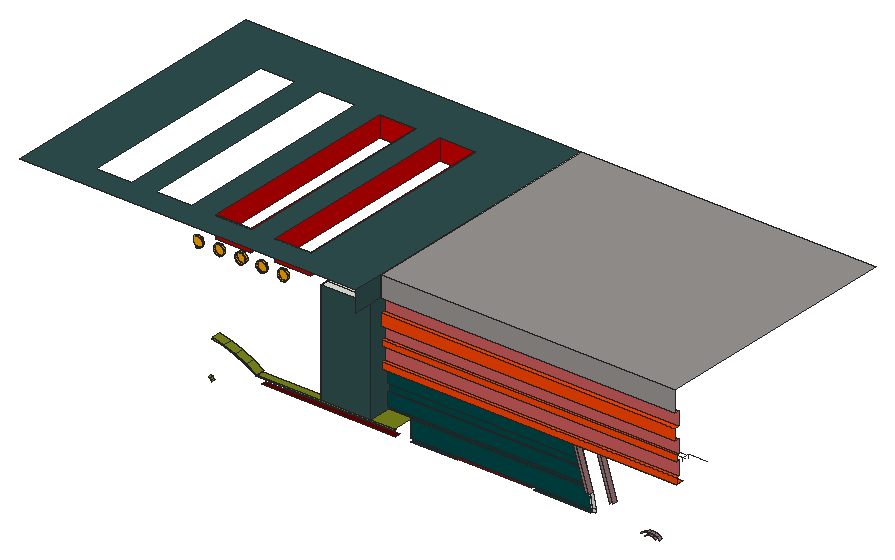
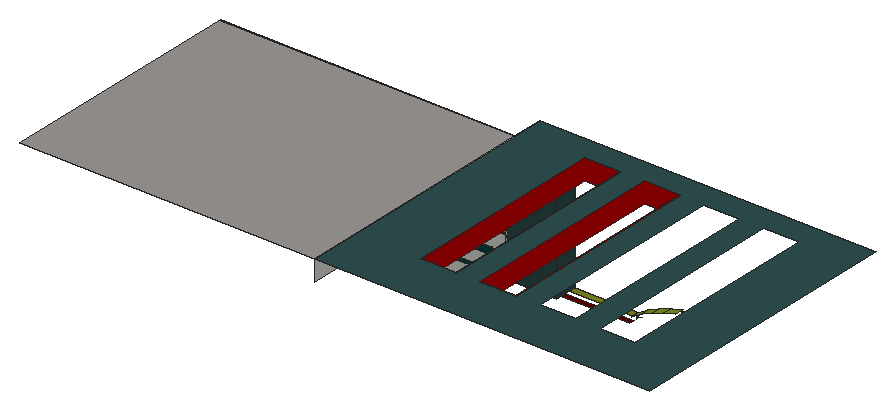
# SketchUp Ruby script. Lengths in inches.
U = 1.inch
M = Sketchup.active_model
def pt(a) = Geom::Point3d.new(a.map { |v| v * U })
def face(e, loops, mat)
  f = e.add_face(loops[0].map { |a| pt(a) })
  loops[1..].each { |l| e.add_face(l.map { |a| pt(a) }).erase! }
  f.material = f.back_material = mat if mat
  f
end
# faces: each face lists its corners as indices into pts; further lists are holes
def faces(e, pts, list, mat = nil) = list.each { |f| face(e, (f[0].is_a?(Array) ? f : [f]).map { |l| l.map { |i| pts[i] } }, mat) }
# xy, xz, yz: faces in a plane at the given z, y or x. An outline is a flat list of corners, or four numbers for a rectangle; further outlines are holes
def ring(l) = l.size == 4 ? [[l[0], l[1]], [l[2], l[1]], [l[2], l[3]], [l[0], l[3]]] : l.each_slice(2).to_a
def flat(e, list, mat, &to3) = list.each { |f| face(e, (f[0].is_a?(Array) ? f : [f]).map { |l| ring(l).map { |u, v| to3.(u, v) } }, mat) }
def xy(e, z, list, mat = nil) = flat(e, list, mat) { |x, y| [x, y, z] }
def xz(e, y, list, mat = nil) = flat(e, list, mat) { |x, z| [x, y, z] }
def yz(e, x, list, mat = nil) = flat(e, list, mat) { |y, z| [x, y, z] }
def lines(e, pts, list) = list.each { |a, b| e.add_line(pt(pts[a]), pt(pts[b])) }
# prism: a flat outline (further loops are holes) pulled along v
def prism(e, loops, v, mat = nil)
  f = face(e, loops, mat); d = Geom::Vector3d.new(v.map { |x| x * U })
  f.pushpull(f.normal.samedirection?(d) ? d.length : -d.length)
end
def box(e, o, s, mat = nil) = prism(e, [[o, [o[0] + s[0], o[1], o[2]], [o[0] + s[0], o[1] + s[1], o[2]], [o[0], o[1] + s[1], o[2]]]], [0, 0, s[2]], mat)
def at(x, y, z, deg = 0) = Geom::Transformation.translation(pt([x, y, z])) * Geom::Transformation.rotation(ORIGIN, Z_AXIS, deg.degrees)
def axes(o, x, y, z) = Geom::Transformation.new([*x, 0, *y, 0, *z, 0, *pt(o).to_a, 1])
def part(name) = M.definitions.add(name)
# library, detail: a bought-in or finely detailed component or shape, given as its bounding box
def library(name, o, s) = part(name).tap { |d| box(d.entities, o, s) }
def detail(e, o, s) = box(e.add_group.entities, o, s)
def put(e, d, t, mat = nil) = e.add_instance(d, t).tap { |i| i.material = mat if mat }
def group(e, t, mat = nil) = e.add_group.tap { |g| g.transformation = t; g.material = mat if mat }.entities
root = M.entities
M.materials.add("[0017_IndianRed]").color = [205, 92, 92]
M.materials.add("[0020_Red]").color = [165, 0, 0]
M.materials.add("[0020_Red]1").color = [204, 0, 0]
M.materials.add("[0022_Maroon]").color = [99, 0, 0]
M.materials.add("[0024_OrangeRed]").color = [255, 69, 0]
M.materials.add("[0038_Orange]1").color = [255, 165, 0]
M.materials.add("[0057_DarkKhaki]").color = [122, 132, 27]
M.materials.add("[0078_DarkSlateGray]").color = [47, 79, 79]
M.materials.add("[0119_RosyBrown]").color = [150, 114, 114]
M.materials.add("[Color H08]").color = [0, 71, 71]
M.materials.add("[Concrete Aggregate Smoke]").color = [154, 150, 148]
xy(root,288.67,[[221.0625,650.11,247.97,651.11],[292.45,650.11,325.55,651.11]],"[Color H08]")
xy(root,290.61,[[247.97,650.11,292.45,651.11],[247.97,651.11,292.45,656.36]])
xy(root,290.61,[[247.97,648.11,292.45,650.11]],"[0020_Red]")
xy(root,290.61,[[221.0625,650.11,247.97,651.11],[292.45,650.11,325.22,651.11]],"[Color H08]")
xy(root,296.25,[[143.09,639.11,221.0625,642.11]],"[0022_Maroon]")
xy(root,299.9,[[140.36,638.11,221.0625,639.11]],"[0057_DarkKhaki]")
xy(root,300.74,[[178.3125,638.05,207.0625,638.11],[178.3125,638.11,207.0625,642.11],[178.3125,642.11,178.3125,651.24,207.9375,651.24,207.9375,651.11,207.0625,651.11,207.0625,642.11],[207.9375,651.11,221.0625,651.24]])
xy(root,300.74,[[141.15,638.11,178.3125,642.11],[207.0625,638.11,221.0625,651.11]],"[0057_DarkKhaki]")
xy(root,300.74,[[221.0625,650.11,323.2,651.11]],"[Color H08]")
xy(root,302.39,[[207.0625,650.11,207.9375,651.11]])
xy(root,302.39,[[207.9375,650.11,322.69,651.11]],"[Color H08]")
xy(root,310.14,[[207.0625,650.11,320.31,651.11]],"[Color H08]")
xy(root,314.28,[[207.0625,650.11,319.04,651.11]],"[Color H08]")
xy(root,323.31,[[316.26,648.11,317.96,651.11],[207.9375,650.11,316.26,651.11]])
xy(root,323.31,[[207.0625,646.43,207.0625,650.11,316.26,650.11,316.26,648.11,317.96,648.11,317.96,651.11,330.34,651.11,330.34,648.11,332.04,648.11,332.04,651.11,377.9375,651.11,377.9375,646.43]],"[0024_OrangeRed]")
xy(root,326.96,[[207.0625,646.43,377.9375,648.43]],"[0024_OrangeRed]")
xy(root,335.1875,[[207.0625,646.43,377.9375,648.43]],"[0024_OrangeRed]")
xy(root,338.52,[[207.0625,646.43,377.9375,648.43]],"[0024_OrangeRed]")
xy(root,346.17,[[207.0625,645.43,377.9375,648.43]],"[0024_OrangeRed]")
xy(root,352.6875,[[207.0625,645.43,377.9375,648.43]],"[0024_OrangeRed]")
xy(root,360.74,[[178.3125,638.05,207,638.11],[207,638.05,207.0625,645.43],[178.3125,638.11,207,642.11],[178.3125,642.11,207,651.24],[207,645.43,207.0625,645.43,207.0625,648.43,207.9375,648.43,207.9375,651.24,207,651.24]])
xy(root,360.74,[[207.0625,645.43,377.9375,648.43]],"[Concrete Aggregate Smoke]")
xy(root,372.74,[[[12.25,627.18,207,791.05],[45.02,641.59,65.77,760.78],[79.64,641.59,100.39,760.78],[114.27,641.59,135.02,760.78],[148.89,641.59,169.64,760.78]]],"[0078_DarkSlateGray]")
xy(root,372.74,[[207,645.43,377.9375,791.05]],"[Concrete Aggregate Smoke]")
xz(root,628.18,[[115.26,362.59,116.05,362.69,116.79,363,117.42,363.48,117.91,364.12,118.22,364.86,118.32,365.65,118.22,366.44,117.91,367.18,117.42,367.82,116.79,368.3,116.05,368.61,115.26,368.71,114.47,368.61,113.73,368.3,113.09,367.82,112.61,367.18,112.3,366.44,112.2,365.65,112.3,364.86,112.61,364.12,113.09,363.48,113.73,363,114.47,362.69],[127.63,362.59,128.43,362.69,129.16,363,129.8,363.48,130.29,364.12,130.59,364.86,130.7,365.65,130.59,366.44,130.29,367.18,129.8,367.82,129.16,368.3,128.43,368.61,127.63,368.71,126.84,368.61,126.1,368.3,125.47,367.82,124.98,367.18,124.68,366.44,124.57,365.65,124.68,364.86,124.98,364.12,125.47,363.48,126.1,363,126.84,362.69],[152.38,362.59,153.18,362.69,153.91,363,154.55,363.48,155.04,364.12,155.34,364.86,155.45,365.65,155.34,366.44,155.04,367.18,154.55,367.82,153.91,368.3,153.18,368.61,152.38,368.71,151.59,368.61,150.85,368.3,150.22,367.82,149.73,367.18,149.43,366.44,149.32,365.65,149.43,364.86,149.73,364.12,150.22,363.48,150.85,363,151.59,362.69],[164.76,362.59,165.55,362.69,166.29,363,166.92,363.48,167.41,364.12,167.72,364.86,167.82,365.65,167.72,366.44,167.41,367.18,166.92,367.82,166.29,368.3,165.55,368.61,164.76,368.71,163.97,368.61,163.23,368.3,162.59,367.82,162.11,367.18,161.8,366.44,161.7,365.65,161.8,364.86,162.11,364.12,162.59,363.48,163.23,363,163.97,362.69]],"[0038_Orange]1")
xz(root,628.86,[[140.01,362.59,140.8,362.69,141.54,363,142.17,363.48,142.66,364.12,142.97,364.86,143.07,365.65,142.97,366.44,142.66,367.18,142.17,367.82,141.54,368.3,140.8,368.61,140.01,368.71,139.22,368.61,138.48,368.3,137.84,367.82,137.36,367.18,137.05,366.44,136.95,365.65,137.05,364.86,137.36,364.12,137.84,363.48,138.48,363,139.22,362.69]],"[0038_Orange]1")
xz(root,638.05,[[178.3125,300.74,207.0625,360.74]],"[0078_DarkSlateGray]")
xz(root,641.59,[[114.27,360.74,135.02,372.74],[148.89,360.74,169.64,372.74]],"[0020_Red]1")
xz(root,642.11,[[138.39,300.67,141.15,300.6875],[138.39,300.6875,138.39,300.74,138.48,300.6875],[138.48,300.6875,138.39,300.74,141.15,300.74,141.15,300.6875]])
xz(root,645.43,[[207.0625,346.17,377.9375,352.6875]],"[0024_OrangeRed]")
xz(root,645.43,[[207,360.74,377.9375,372.74]],"[Concrete Aggregate Smoke]")
xz(root,646.43,[[207.0625,323.31,377.9375,326.96],[207.0625,335.1875,377.9375,338.52]],"[0024_OrangeRed]")
xz(root,648.43,[[207.9375,335.1875,367,338.52]])
xz(root,648.43,[[207.0625,326.96,377.9375,335.1875],[207.0625,338.52,377.9375,346.17],[207.0625,352.6875,377.9375,360.74]],"[0017_IndianRed]")
xz(root,650.11,[[221.0625,290.61,325.22,290.61,323.87,298.58,323.2,300.74,221.0625,300.74],[207.0625,302.39,322.69,302.39,320.31,310.14,207.0625,310.14],[207.0625,314.28,319.04,314.28,316.26,323.31,207.0625,323.31]],"[Color H08]")
xz(root,651.11,[[325.55,288.67,327.54,288.67,327.19,290.61,325.22,290.61],[221.0625,290.61,221.0625,300.74,323.2,300.74,323.87,298.58,325.22,290.61],[325.22,290.61,327.19,290.61,325.7,298.89,325.11,300.74,323.2,300.74,323.87,298.58],[323.2,300.74,325.11,300.74,324.59,302.39,322.69,302.39],[207.9375,302.39,207.9375,310.14,320.31,310.14,322.69,302.39],
  [322.69,302.39,324.59,302.39,322.13,310.14,320.31,310.14],[320.31,310.14,322.13,310.14,319.04,319.9,319.04,314.28],[207.9375,314.28,207.9375,323.31,316.26,323.31,319.04,314.28],[319.04,314.28,319.04,319.9,317.96,323.31,316.26,323.31]])
xz(root,651.11,[[221.0625,288.67,247.97,290.61],[292.45,288.67,325.55,288.67,325.22,290.61,292.45,290.61],[207.0625,300.74,323.2,300.74,322.69,302.39,207.0625,302.39],[207.0625,310.14,320.31,310.14,319.04,314.28,207.0625,314.28]],"[Color H08]")
xz(root,651.24,[[207,300.74,207.9375,360.74]])
xz(root,651.24,[[178.3125,300.74,207,360.74]],"[0078_DarkSlateGray]")
xz(root,760.78,[[114.27,360.74,135.02,372.74],[148.89,360.74,169.64,372.74]],"[0020_Red]1")
yz(root,114.27,[[641.59,360.74,760.78,372.74]],"[0020_Red]1")
yz(root,135.02,[[641.59,360.74,760.78,372.74]],"[0020_Red]1")
yz(root,140.36,[[638.11,299.9,639.11,300.29]],"[0057_DarkKhaki]")
yz(root,141.15,[[639.11,300.67,642.11,300.6875],[642.11,300.67,643.36,300.6875],[639.11,300.6875,642.11,300.74],[642.11,300.6875,643.36,300.74]])
yz(root,148.89,[[641.59,360.74,760.78,372.74]],"[0020_Red]1")
yz(root,169.64,[[641.59,360.74,760.78,372.74]],"[0020_Red]1")
yz(root,178.3125,[[638.05,300.74,651.24,360.74]],"[0078_DarkSlateGray]")
yz(root,207,[[645.43,360.74,791.05,372.74]])
yz(root,207,[[627.18,360.74,645.43,372.74]],"[0078_DarkSlateGray]")
yz(root,207.0625,[[638.05,300.74,651.11,300.74,651.11,302.39,650.11,302.39,650.11,310.14,651.11,310.14,651.11,314.28,650.11,314.28,650.11,323.31,646.43,323.31,646.43,326.96,648.43,326.96,648.43,335.1875,646.43,335.1875,646.43,338.52,648.43,338.52,648.43,346.17,645.43,346.17,645.43,352.6875,648.43,352.6875,648.43,360.74,638.05,360.74]],"[0078_DarkSlateGray]")
yz(root,221.0625,[[650.11,290.61,651.11,300.74]])
yz(root,247.97,[[651.11,288.67,656.36,290.61]])
yz(root,292.45,[[651.11,288.67,656.36,290.61]])
p = [[357.6875,651.11,288.52],[359.11,651.11,289.11],[359.11,649.11,289.11],[357.6875,649.11,288.52],[362.16,651.11,289.11],[363.58,651.11,288.52],
  [363.58,649.11,288.52],[362.16,649.11,289.11],[115.7,639.11,288.64],[115.4,639.11,289.31],[115.4,637.11,289.31],[115.7,637.11,288.64],
  [356.85,651.11,289.97],[355.29,651.11,288.77],[355.29,649.11,288.77],[356.85,649.11,289.97],[365.98,651.11,288.77],[364.42,651.11,289.97],
  [364.42,649.11,289.97],[365.98,649.11,288.77],[360.63,651.11,289.3125],[360.63,649.11,289.3125],[114.97,639.11,289.9],[114.97,637.11,289.9],
  [114.43,639.11,290.38],[114.43,637.11,290.38],[358.68,651.11,290.72],[358.68,649.11,290.72],[362.59,651.11,290.72],[362.59,649.11,290.72],
  [113.8,639.11,290.75],[113.8,637.11,290.75],[323.87,651.11,298.58],[325.22,651.11,290.61],[325.22,650.11,290.61],[323.87,650.11,298.58],
  [360.63,651.11,290.98],[360.63,649.11,290.98],[322.69,651.11,302.39],[323.2,651.11,300.74],[323.2,650.11,300.74],[323.87,648.11,298.58],
  [316.26,648.11,323.31],[316.26,650.11,323.31],[319.04,650.11,314.28],[319.04,651.11,314.28],[320.31,651.11,310.14],[320.31,650.11,310.14],
  [322.69,650.11,302.39],[330.34,651.11,323.31],[337.94,651.11,298.58],[337.94,648.11,298.58],[330.34,648.11,323.31],[325.7,651.11,298.89],
  [325.11,651.11,300.74],[324.59,651.11,302.39],[322.13,651.11,310.14],[319.04,651.11,319.9],[317.96,651.11,323.31],[317.96,648.11,323.31],
  [325.7,648.11,298.89],[339.78,651.11,298.89],[332.04,651.11,323.31],[332.04,648.11,323.31],[339.78,648.11,298.89],[134.72,639.11,303.6],
  [140.36,639.11,300.29],[140.36,638.11,300.29],[134.72,638.11,303.6],[135.09,643.36,304.29],[135.09,638.11,304.29],[141.15,638.11,300.74],
  [141.15,639.11,300.74],[141.15,642.11,300.74],[141.15,643.36,300.74],[128.42,639.11,306.52],[128.42,638.11,306.52],[128.71,643.36,307.25],
  [128.71,638.11,307.25],[121.85,639.11,308.82],[121.85,638.11,308.82],[122.08,643.36,309.58],[122.08,638.11,309.58],[115.1,639.11,310.48],
  [115.1,638.11,310.48],[115.25,643.36,311.26],[115.25,638.11,311.26],[316.26,651.11,323.31],[114.47,627.18,362.69],[115.26,627.18,362.59],
  [115.26,628.18,362.59],[114.47,628.18,362.69],[116.05,627.18,362.69],[116.05,628.18,362.69],[126.84,627.18,362.69],[127.63,627.18,362.59],
  [127.63,628.18,362.59],[126.84,628.18,362.69],[128.43,627.18,362.69],[128.43,628.18,362.69],[139.22,627.18,362.69],[140.01,627.18,362.59],
  [140.01,627.24,362.59],[139.22,627.24,362.69],[139.22,628.86,362.69],[140.01,628.86,362.59],[140.8,627.18,362.69],[140.8,627.24,362.69],
  [140.8,628.86,362.69],[151.59,627.18,362.69],[152.38,627.18,362.59],[152.38,628.18,362.59],[151.59,628.18,362.69],[153.18,627.18,362.69],
  [153.18,628.18,362.69],[163.97,627.18,362.69],[164.76,627.18,362.59],[164.76,628.18,362.59],[163.97,628.18,362.69],[165.55,627.18,362.69],
  [165.55,628.18,362.69],[116.79,627.18,363],[116.79,628.18,363],[126.1,627.18,363],[126.1,628.18,363],[129.16,627.18,363],
  [129.16,628.18,363],[138.48,627.18,363],[138.48,627.24,363],[138.48,628.86,363],[141.54,627.18,363],[141.54,627.24,363],
  [141.54,628.86,363],[150.85,627.18,363],[150.85,628.18,363],[153.91,627.18,363],[153.91,628.18,363],[163.23,627.18,363],
  [163.23,628.18,363],[166.29,627.18,363],[166.29,628.18,363],[117.42,627.18,363.48],[117.42,628.18,363.48],[125.47,627.18,363.48],
  [125.47,628.18,363.48],[129.8,627.18,363.48],[129.8,628.18,363.48],[137.84,627.18,363.48],[137.84,627.24,363.48],[137.84,628.86,363.48],
  [142.17,627.18,363.48],[142.17,627.24,363.48],[142.17,628.86,363.48],[150.22,627.18,363.48],[150.22,628.18,363.48],[154.55,627.18,363.48],
  [154.55,628.18,363.48],[162.59,627.18,363.48],[162.59,628.18,363.48],[166.92,627.18,363.48],[166.92,628.18,363.48],[117.91,627.18,364.12],
  [117.91,628.18,364.12],[124.98,627.18,364.12],[124.98,628.18,364.12],[130.29,627.18,364.12],[130.29,628.18,364.12],[137.36,627.18,364.12],
  [137.36,627.24,364.12],[137.36,628.86,364.12],[142.66,627.18,364.12],[142.66,627.24,364.12],[142.66,628.86,364.12],[149.73,627.18,364.12],
  [149.73,628.18,364.12],[155.04,627.18,364.12],[155.04,628.18,364.12],[162.11,627.18,364.12],[162.11,628.18,364.12],[167.41,627.18,364.12],
  [167.41,628.18,364.12],[118.22,627.18,364.86],[118.22,628.18,364.86],[124.68,627.18,364.86],[124.68,628.18,364.86],[130.59,627.18,364.86],
  [130.59,628.18,364.86],[137.05,627.18,364.86],[137.05,627.24,364.86],[137.05,628.86,364.86],[142.97,627.18,364.86],[142.97,627.24,364.86],
  [142.97,628.86,364.86],[149.43,627.18,364.86],[149.43,628.18,364.86],[155.34,627.18,364.86],[155.34,628.18,364.86],[161.8,627.18,364.86],
  [161.8,628.18,364.86],[167.72,627.18,364.86],[167.72,628.18,364.86],[118.32,627.18,365.65],[118.32,628.18,365.65],[124.57,627.18,365.65],
  [124.57,628.18,365.65],[130.7,627.18,365.65],[130.7,628.18,365.65],[136.95,627.18,365.65],[136.95,627.24,365.65],[136.95,628.86,365.65],
  [143.07,627.18,365.65],[143.07,627.24,365.65],[143.07,628.86,365.65],[149.32,627.18,365.65],[149.32,628.18,365.65],[155.45,627.18,365.65],
  [155.45,628.18,365.65],[161.7,627.18,365.65],[161.7,628.18,365.65],[167.82,627.18,365.65],[167.82,628.18,365.65],[118.22,627.18,366.44],
  [118.22,628.18,366.44],[124.68,627.18,366.44],[124.68,628.18,366.44],[130.59,627.18,366.44],[130.59,628.18,366.44],[137.05,627.18,366.44],
  [137.05,627.24,366.44],[137.05,628.86,366.44],[142.97,627.18,366.44],[142.97,627.24,366.44],[142.97,628.86,366.44],[149.43,627.18,366.44],
  [149.43,628.18,366.44],[155.34,627.18,366.44],[155.34,628.18,366.44],[161.8,627.18,366.44],[161.8,628.18,366.44],[167.72,627.18,366.44],
  [167.72,628.18,366.44],[117.91,627.18,367.18],[117.91,628.18,367.18],[124.98,627.18,367.18],[124.98,628.18,367.18],[130.29,627.18,367.18],
  [130.29,628.18,367.18],[137.36,627.18,367.18],[137.36,627.24,367.18],[137.36,628.86,367.18],[142.66,627.18,367.18],[142.66,627.24,367.18],
  [142.66,628.86,367.18],[149.73,627.18,367.18],[149.73,628.18,367.18],[155.04,627.18,367.18],[155.04,628.18,367.18],[162.11,627.18,367.18],
  [162.11,628.18,367.18],[167.41,627.18,367.18],[167.41,628.18,367.18],[117.42,627.18,367.82],[117.42,628.18,367.82],[125.47,627.18,367.82],
  [125.47,628.18,367.82],[129.8,627.18,367.82],[129.8,628.18,367.82],[137.84,627.18,367.82],[137.84,627.24,367.82],[137.84,628.86,367.82],
  [142.17,627.18,367.82],[142.17,627.24,367.82],[142.17,628.86,367.82],[150.22,627.18,367.82],[150.22,628.18,367.82],[154.55,627.18,367.82],
  [154.55,628.18,367.82],[162.59,627.18,367.82],[162.59,628.18,367.82],[166.92,627.18,367.82],[166.92,628.18,367.82],[116.79,627.18,368.3],
  [116.79,628.18,368.3],[126.1,627.18,368.3],[126.1,628.18,368.3],[129.16,627.18,368.3],[129.16,628.18,368.3],[138.48,627.18,368.3],
  [138.48,627.24,368.3],[138.48,628.86,368.3],[141.54,627.18,368.3],[141.54,627.24,368.3],[141.54,628.86,368.3],[150.85,627.18,368.3],
  [150.85,628.18,368.3],[153.91,627.18,368.3],[153.91,628.18,368.3],[163.23,627.18,368.3],[163.23,628.18,368.3],[166.29,627.18,368.3],
  [166.29,628.18,368.3],[116.05,627.18,368.61],[116.05,628.18,368.61],[126.84,627.18,368.61],[126.84,628.18,368.61],[128.43,627.18,368.61],
  [128.43,628.18,368.61],[139.22,627.18,368.61],[139.22,627.24,368.61],[139.22,628.86,368.61],[140.8,627.18,368.61],[140.8,627.24,368.61],
  [140.8,628.86,368.61],[151.59,627.18,368.61],[151.59,628.18,368.61],[153.18,627.18,368.61],[153.18,628.18,368.61],[163.97,627.18,368.61],
  [163.97,628.18,368.61],[165.55,627.18,368.61],[165.55,628.18,368.61],[115.26,627.18,368.71],[114.47,627.18,368.61],[114.47,628.18,368.61],
  [115.26,628.18,368.71],[127.63,627.18,368.71],[127.63,628.18,368.71],[140.01,627.18,368.71],[140.01,627.24,368.71],[140.01,628.86,368.71],
  [152.38,627.18,368.71],[152.38,628.18,368.71],[164.76,627.18,368.71],[164.76,628.18,368.71],[138.48,640.93,300.6875],[141.15,640.93,300.6875],
  [136.01,642.18,302.13],[136.01,643.36,302.13],[138.39,642.18,300.74],[138.39,643.36,300.74],[367,664.61,323.31],[367,664.61,325.46],
  [207.9375,648.43,323.31],[207.9375,648.43,326.96],[367,668.8,323.375],[367,668.8,325.46],[367,652.61,334.1875],[367,652.61,336.27],
  [367,648.43,336.27],[367,648.43,334.1875],[377.9375,652.61,336.27],[377.9375,652.61,334.1875],[377.9375,668.8,325.46],[377.9375,648.43,323.375],
  [377.9375,648.43,323.31]]
faces(root,p,[[0,1,2,3],[4,5,6,7],[12,13,14,15],[16,17,18,19],[1,20,21,2],[20,4,7,21],[26,12,15,27],[17,28,29,18],
  [36,26,27,37],[28,36,37,29],[38,39,40,35,41,42,43,44,45,46,47,48],[49,50,51,52],[53,54,55,56,57,58,59,60],[61,62,63,64]],"[0119_RosyBrown]")
faces(root,p,[[8,9,10,11],[9,22,23,10],[22,24,25,23],[24,30,31,25],[65,66,67,68],[69,70,71,72,73,74],[75,65,68,76],[77,78,70,69],
  [79,75,76,80],[81,82,78,77],[83,79,80,84],[85,86,82,81]],"[0057_DarkKhaki]")
faces(root,p,[[32,33,34,35],[39,32,35,40],[46,38,48,47],[87,45,44,43],[100,101,102,103],[101,106,107,102],[127,100,103,128],[106,130,131,107],
  [147,127,128,148],[130,150,151,131],[167,147,148,168],[150,170,171,151],[187,167,168,188],[170,190,191,171],[207,187,188,208],[190,210,211,191],
  [227,207,208,228],[210,230,231,211],[247,227,228,248],[230,250,251,231],[267,247,248,268],[250,270,271,251],[287,267,268,288],[270,290,291,271],
  [307,287,288,308],[290,310,311,291],[327,307,308,328],[310,327,328,311]])
faces(root,p,[[88,89,90,91],[89,92,93,90],[94,95,96,97],[95,98,99,96],[104,103,102,105],[105,102,107,108],[109,110,111,112],[110,113,114,111],
  [115,116,117,118],[116,119,120,117],[92,121,122,93],[123,94,97,124],[98,125,126,99],[129,128,103,104],[108,107,131,132],[133,109,112,134],
  [113,135,136,114],[137,115,118,138],[119,139,140,120],[121,141,142,122],[143,123,124,144],[125,145,146,126],[149,148,128,129],[132,131,151,152],
  [153,133,134,154],[135,155,156,136],[157,137,138,158],[139,159,160,140],[141,161,162,142],[163,143,144,164],[145,165,166,146],[169,168,148,149],
  [152,151,171,172],[173,153,154,174],[155,175,176,156],[177,157,158,178],[159,179,180,160],[161,181,182,162],[183,163,164,184],[165,185,186,166],
  [189,188,168,169],[172,171,191,192],[193,173,174,194],[175,195,196,176],[197,177,178,198],[179,199,200,180],[181,201,202,182],[203,183,184,204],
  [185,205,206,186],[209,208,188,189],[192,191,211,212],[213,193,194,214],[195,215,216,196],[217,197,198,218],[199,219,220,200],[201,221,222,202],
  [223,203,204,224],[205,225,226,206],[229,228,208,209],[212,211,231,232],[233,213,214,234],[215,235,236,216],[237,217,218,238],[219,239,240,220],
  [221,241,242,222],[243,223,224,244],[225,245,246,226],[249,248,228,229],[232,231,251,252],[253,233,234,254],[235,255,256,236],[257,237,238,258],
  [239,259,260,240],[241,261,262,242],[263,243,244,264],[245,265,266,246],[269,268,248,249],[252,251,271,272],[273,253,254,274],[255,275,276,256],
  [277,257,258,278],[259,279,280,260],[261,281,282,262],[283,263,264,284],[265,285,286,266],[289,288,268,269],[272,271,291,292],[293,273,274,294],
  [275,295,296,276],[297,277,278,298],[279,299,300,280],[281,301,302,282],[303,283,284,304],[285,305,306,286],[309,308,288,289],[292,291,311,312],
  [313,293,294,314],[295,315,316,296],[317,297,298,318],[299,319,320,300],[321,322,323,324],[301,321,324,302],[325,303,304,326],[305,325,326,306],
  [329,328,308,309],[312,311,328,329],[330,313,314,331],[315,330,331,316],[332,317,318,333],[319,332,333,320]],"[0038_Orange]1")
lines(root,p,[[334,335],[336,337],[338,339],[340,341],[342,343],[344,345],[341,345],[346,347],[348,347],[349,346],[347,350],[346,351],
  [345,352],[353,354]])
